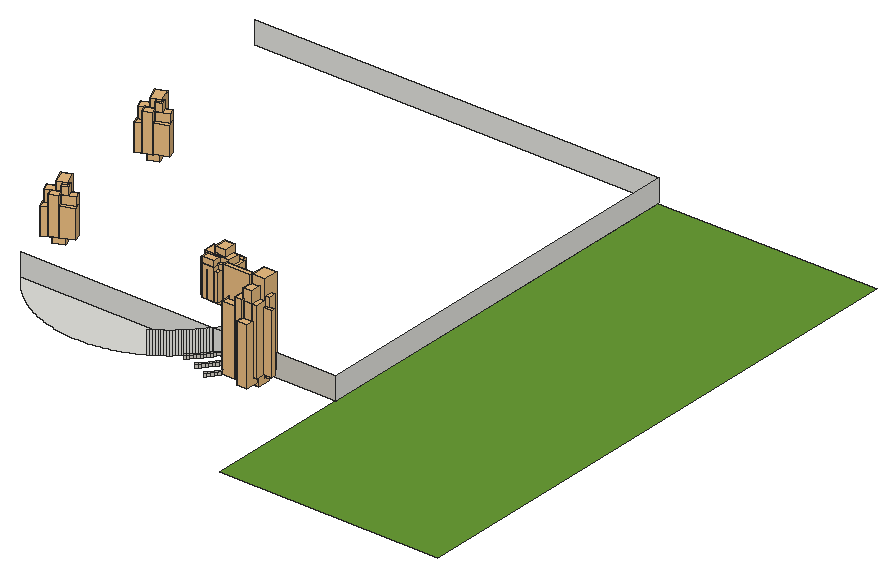
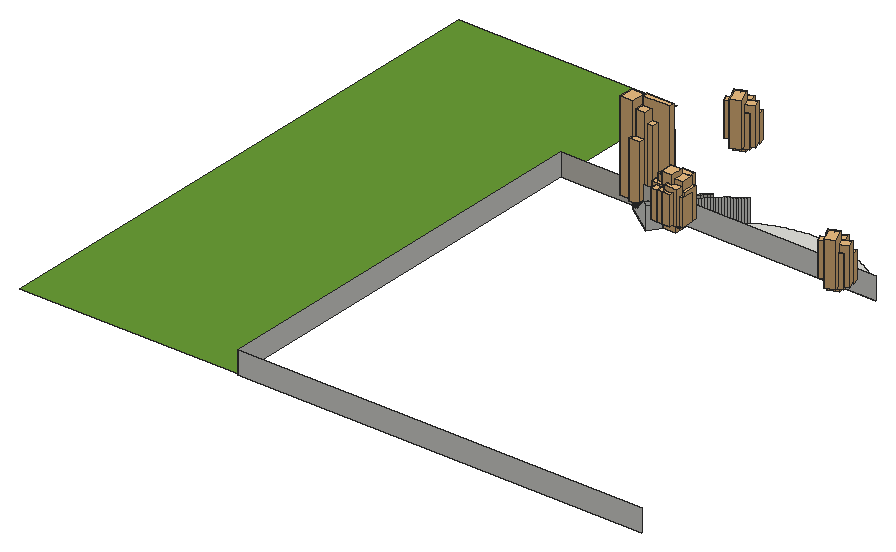
# SketchUp Ruby script. Lengths in inches.
U = 1.inch
M = Sketchup.active_model
def pt(a) = Geom::Point3d.new(a.map { |v| v * U })
def face(e, loops, mat)
  f = e.add_face(loops[0].map { |a| pt(a) })
  loops[1..].each { |l| e.add_face(l.map { |a| pt(a) }).erase! }
  f.material = f.back_material = mat if mat
  f
end
# faces: each face lists its corners as indices into pts; further lists are holes
def faces(e, pts, list, mat = nil) = list.each { |f| face(e, (f[0].is_a?(Array) ? f : [f]).map { |l| l.map { |i| pts[i] } }, mat) }
# xy, xz, yz: faces in a plane at the given z, y or x. An outline is a flat list of corners, or four numbers for a rectangle; further outlines are holes
def ring(l) = l.size == 4 ? [[l[0], l[1]], [l[2], l[1]], [l[2], l[3]], [l[0], l[3]]] : l.each_slice(2).to_a
def flat(e, list, mat, &to3) = list.each { |f| face(e, (f[0].is_a?(Array) ? f : [f]).map { |l| ring(l).map { |u, v| to3.(u, v) } }, mat) }
def xy(e, z, list, mat = nil) = flat(e, list, mat) { |x, y| [x, y, z] }
def xz(e, y, list, mat = nil) = flat(e, list, mat) { |x, z| [x, y, z] }
def yz(e, x, list, mat = nil) = flat(e, list, mat) { |y, z| [x, y, z] }
def lines(e, pts, list) = list.each { |a, b| e.add_line(pt(pts[a]), pt(pts[b])) }
# prism: a flat outline (further loops are holes) pulled along v
def prism(e, loops, v, mat = nil)
  f = face(e, loops, mat); d = Geom::Vector3d.new(v.map { |x| x * U })
  f.pushpull(f.normal.samedirection?(d) ? d.length : -d.length)
end
def box(e, o, s, mat = nil) = prism(e, [[o, [o[0] + s[0], o[1], o[2]], [o[0] + s[0], o[1] + s[1], o[2]], [o[0], o[1] + s[1], o[2]]]], [0, 0, s[2]], mat)
def at(x, y, z, deg = 0) = Geom::Transformation.translation(pt([x, y, z])) * Geom::Transformation.rotation(ORIGIN, Z_AXIS, deg.degrees)
def axes(o, x, y, z) = Geom::Transformation.new([*x, 0, *y, 0, *z, 0, *pt(o).to_a, 1])
def part(name) = M.definitions.add(name)
# library, detail: a bought-in or finely detailed component or shape, given as its bounding box
def library(name, o, s) = part(name).tap { |d| box(d.entities, o, s) }
def detail(e, o, s) = box(e.add_group.entities, o, s)
def put(e, d, t, mat = nil) = e.add_instance(d, t).tap { |i| i.material = mat if mat }
def group(e, t, mat = nil) = e.add_group.tap { |g| g.transformation = t; g.material = mat if mat }.entities
root = M.entities
M.materials.add("Arta-Ceramic-Moonstone-White-24x24-4K").color = [209, 205, 196]
M.materials.add("POT_TEXTURE_1").color = [172, 172, 172]
M.materials.add("[Grass Dark Green]").color = [106, 157, 55]
M.materials.add("soil1").color = [68, 55, 47]
M.materials.add("white_concrete_pot1").color = [212, 211, 204]
c1 = library("Group\#13",[-312.76,2118.02,370.79],[80.37,61.43,57.53])
c2 = library("Group\#34",[-146.29,2044.53,349.125],[81,53.32,37.9])
c3 = library("Group\#80",[-236.03,2064.57,238.29],[378.97,266.89,1422.96])
c4 = library("Group\#22",[-392.38,2142.99,345.23],[79.77,60.6,39.05])
c5 = library("Group\#49",[-390.04,2074.71,363.78],[77.3,84.83,61.55])
c6 = library("Group\#26",[-389.63,2051.04,359.41],[56.81,81.38,37.86])
c7 = library("Group\#30",[-362.86,1963.26,351.01],[55.56,80.44,37.9])
c8 = library("Group\#33",[-200.52,1998.86,370.22],[77.15,68.38,35.39])
c9 = library("Group\#45",[-480.58,1843.32,11.96],[467.85,466.24,378.92])
c10 = library("Group\#23",[-433.57,2042.61,369.7],[71.79,72.8,37.85])
c11 = library("Group\#20",[-148.5,2084.1,354.63],[73.89,71.73,39.48])
c12 = library("Group\#62",[-372.4375,2154.5,374],[76.125,67.08,39.0625])
c13 = library("Group\#63",[-275.5,2156.34,352.11],[71.39,73.27,44.69])
c14 = library("Group\#39",[-143.56,2061.14,371.42],[79.79,63.19,51.3])
c15 = library("Group\#48",[-363.89,1895.22,354.63],[76.92,66.54,39.48])
c16 = library("Group\#41",[-145.08,2015.32,369.99],[82.29,54.05,37.9])
c17 = library("Group\#59",[-315.77,2202.04,371],[80.74,54.44,37.85])
c18 = library("Group\#50",[-419.21,1941.11,355.02],[73.1,71.21,39.06])
c19 = library("Group\#53",[-229.79,1894.04,351.01],[79.82,63.55,37.9])
c20 = library("Group\#67",[-234.26,2180.97,367.05],[50.63,74.65,43.95])
c21 = library("Group\#69",[-904.81,1865.01,156.3],[624.43,217.34,1227.7])
c22 = library("Group\#70",[-312.51,1611.52,263.78],[120.52,408.52,1275.1])
c23 = library("Group\#71",[-571.16,1736.08,232.33],[294.08,306.57,1438.75])
c24 = library("Group\#73",[-273.21,1593.22,47.51],[374.54,419.07,1416.6])
c25 = library("Group\#17",[-202.35,1900.5,372.29],[58.53,80.11,50.06])
c26 = library("Group\#25",[-432.01,1984.38,372.6875],[64.1,75.95,39.0625])
c27 = library("Group\#38",[-310.7,1952.62,354.63],[79.53,58.52,39.48])
c28 = library("Group\#24",[-374.28,1979.7,369.99],[51.81,82.66,37.9])
c29 = library("Group\#56",[-397.18,1916.74,372.44],[70.02,74.57,49.25])
c30 = library("Group\#65",[-236.3,2186.8,344.47],[79.26,62.91,39.06])
c31 = library("Group\#16",[-161.07,2117.49,373.61],[81.25,53.73,39.48])
c32 = library("Group\#68",[-431.9,1883.46,368.72],[373.65,376.39,18.61])
c33 = library("Group\#37",[-340.96,1970.4,361.28],[81.22,51.59,61.62])
c34 = library("Group\#43",[-272.7,1884.51,369.99],[80.39,55.87,37.9])
c35 = library("Group\#32",[-330.83,2117.69,370.2],[61.83,80.2,35.55])
c36 = library("Group\#66",[-366.3125,2177.8,359.41],[79.9,61.23,37.86])
c37 = library("Group\#29",[-435.875,2067.96,347.82],[58.32,80.53,38.29])
c38 = library("Group\#64",[-183.79,2161.45,371.25],[72.43,70.21,54.35])
c39 = library("Group\#72",[-208.23,2037.18,75.37],[621.09,225.61,1251.82])
c40 = library("Group\#75",[-675.58,1862.05,152.55],[378.81,196.01,1743.84])
c41 = library("Group\#76",[-257.06,2048.08,160.05],[394.6,177.93,1743.83])
c42 = library("Group\#77",[-344.84,1500.61,160.55],[176.35,551.19,1921.45])
c43 = library("Group\#78",[-231.77,1913.24,119.96],[448.93,143.84,1582.05])
c44 = library("Group\#79",[-616.67,2098.6,178.29],[331.19,111.16,1177.92])
c45 = library("Group\#74",[-527.15,2088.47,150.96],[267.01,328.12,1599.25])
c46 = library("Group\#81",[-792.12,2067.32,152.13],[549.56,259.52,1931.8])
c47 = library("Group\#82",[-281.17,2118.67,243.77],[133.23,408.71,1313.3])
c48 = part("Tall potted plant")
g1 = group(c48.entities,at(904.81,-1500.61,-11.96),"white_concrete_pot1")
detail(g1,[-222.14,2117.95,372.07],[61.87,75.41,50.35])
put(c48.entities,c1,at(904.81,-1500.61,-11.96),"white_concrete_pot1")
g2 = group(c48.entities,at(904.81,-1500.61,-11.96),"white_concrete_pot1")
detail(g2,[-313.93,1881.02,351.21],[70.15,73.18,37.2])
g3 = group(c48.entities,at(904.81,-1500.61,-11.96),"white_concrete_pot1")
detail(g3,[-209.1,1970.26,378.89],[50.57,81.04,37.2])
put(c48.entities,c2,at(904.81,-1500.61,-11.96),"white_concrete_pot1")
put(c48.entities,c3,axes([904.81,-1500.61,-66.4],[1,0,0],[0,1,0],[0,0,2.14595]))
put(c48.entities,c4,at(904.81,-1500.61,-11.96),"white_concrete_pot1")
put(c48.entities,c5,at(904.81,-1500.61,-11.96),"white_concrete_pot1")
put(c48.entities,c6,at(904.81,-1500.61,-11.96),"white_concrete_pot1")
put(c48.entities,c7,at(904.81,-1500.61,-11.96),"white_concrete_pot1")
g4 = group(c48.entities,at(904.81,-1500.61,-11.96),"white_concrete_pot1")
detail(g4,[-129.49,1972.75,359.91],[55.59,80.76,37.2])
put(c48.entities,c8,at(904.81,-1500.61,-11.96),"white_concrete_pot1")
g5 = group(c48.entities,at(904.81,-1500.61,-11.96),"white_concrete_pot1")
detail(g5,[-333.13,1892.25,370.19],[61.39,79.4,37.2])
put(c48.entities,c9,at(904.81,-1500.61,-11.96),"POT_TEXTURE_1")
put(c48.entities,c10,at(904.81,-1500.61,-11.96),"white_concrete_pot1")
put(c48.entities,c11,at(904.81,-1500.61,-11.96),"white_concrete_pot1")
g6 = group(c48.entities,at(904.81,-1500.61,-11.96),"white_concrete_pot1")
detail(g6,[-270.91,2176.57,345.18],[52.11,82.01,38.29])
g7 = group(c48.entities,at(904.81,-1500.61,-11.96),"white_concrete_pot1")
detail(g7,[-195.71,2019.1875,371.11],[58.98,81.18,37.2])
g8 = group(c48.entities,at(904.81,-1500.61,-11.96),"white_concrete_pot1")
detail(g8,[-319.36,2078.81,339.18],[76.07,69.08,39.48])
put(c48.entities,c12,at(904.81,-1500.61,-11.96),"white_concrete_pot1")
put(c48.entities,c13,at(904.81,-1500.61,-11.96),"white_concrete_pot1")
g9 = group(c48.entities,at(904.81,-1500.61,-11.96),"white_concrete_pot1")
detail(g9,[-417.64,2112.53,369.82],[65.44,79.59,38.29])
put(c48.entities,c14,at(904.81,-1500.61,-11.96),"white_concrete_pot1")
put(c48.entities,c15,at(904.81,-1500.61,-11.96),"white_concrete_pot1")
put(c48.entities,c16,at(904.81,-1500.61,-11.96),"white_concrete_pot1")
g10 = group(c48.entities,at(904.81,-1500.61,-11.96),"white_concrete_pot1")
detail(g10,[-240.6,2054.85,378.89],[71.5,72.03,37.2])
put(c48.entities,c17,at(904.81,-1500.61,-11.96),"white_concrete_pot1")
put(c48.entities,c18,at(904.81,-1500.61,-11.96),"white_concrete_pot1")
put(c48.entities,c19,at(904.81,-1500.61,-11.96),"white_concrete_pot1")
g11 = group(c48.entities,at(904.81,-1500.61,-11.96),"white_concrete_pot1")
detail(g11,[-249.82,2117.53,359.91],[58.07,81.25,37.2])
put(c48.entities,c20,at(904.81,-1500.61,-11.96),"white_concrete_pot1")
put(c48.entities,c21,axes([904.81,-1500.61,-66.4],[1,0,0],[0,1,0],[0,0,2.14595]))
put(c48.entities,c22,axes([904.81,-1500.61,-66.4],[1,0,0],[0,1,0],[0,0,2.14595]))
put(c48.entities,c23,axes([904.81,-1500.61,-66.4],[1,0,0],[0,1,0],[0,0,2.14595]))
put(c48.entities,c24,axes([904.81,-1500.61,-66.4],[1,0,0],[0,1,0],[0,0,2.14595]))
g12 = group(c48.entities,at(904.81,-1500.61,-11.96),"white_concrete_pot1")
detail(g12,[-435.4375,2027.54,350.71],[78.74,62.6,37.86])
put(c48.entities,c25,at(904.81,-1500.61,-11.96),"white_concrete_pot1")
g13 = group(c48.entities,at(904.81,-1500.61,-11.96),"white_concrete_pot1")
detail(g13,[-173.8,2126.25,354.63],[80.17,60.53,39.48])
g14 = group(c48.entities,at(904.81,-1500.61,-11.96),"white_concrete_pot1")
detail(g14,[-222.96,2066.75,359.91],[63.77,78.21,37.2])
put(c48.entities,c26,at(904.81,-1500.61,-11.96),"white_concrete_pot1")
g15 = group(c48.entities,at(904.81,-1500.61,-11.96),"white_concrete_pot1")
detail(g15,[-183.125,1913.38,330.04],[66.78,77.69,39.48])
put(c48.entities,c27,at(904.81,-1500.61,-11.96),"white_concrete_pot1")
g16 = group(c48.entities,at(904.81,-1500.61,-11.96),"white_concrete_pot1")
detail(g16,[-152,1936.85,378.89],[64.46,79.76,37.2])
g17 = group(c48.entities,at(904.81,-1500.61,-11.96),"white_concrete_pot1")
detail(g17,[-284.65,1933.22,373.64],[80.83,55.23,37.2])
put(c48.entities,c28,at(904.81,-1500.61,-11.96),"white_concrete_pot1")
g18 = group(c48.entities,at(904.81,-1500.61,-11.96),"white_concrete_pot1")
detail(g18,[-263.49,1923.54,359.91],[75.98,66.75,37.2])
put(c48.entities,c29,at(904.81,-1500.61,-11.96),"white_concrete_pot1")
g19 = group(c48.entities,at(904.81,-1500.61,-11.96),"white_concrete_pot1")
detail(g19,[-167.97,1940.97,354.63],[66.78,77.7,39.48])
put(c48.entities,c30,at(904.81,-1500.61,-11.96),"white_concrete_pot1")
g20 = group(c48.entities,at(904.81,-1500.61,-11.96),"white_concrete_pot1")
detail(g20,[-214.75,1956.59,330.04],[66.78,77.69,39.48])
put(c48.entities,c31,at(904.81,-1500.61,-11.96),"white_concrete_pot1")
put(c48.entities,c32,at(904.81,-1500.61,-11.96),"white_concrete_pot1")
put(c48.entities,c33,at(904.81,-1500.61,-11.96),"white_concrete_pot1")
g21 = group(c48.entities,at(904.81,-1500.61,-11.96),"white_concrete_pot1")
detail(g21,[-282.5625,1934.21,389.56],[81.1,59.19,35.03])
put(c48.entities,c34,at(904.81,-1500.61,-11.96),"white_concrete_pot1")
g22 = group(c48.entities,at(904.81,-1500.61,-11.96),"white_concrete_pot1")
detail(g22,[-394.5,2036.48,359.91],[79.58,64.84,37.2])
put(c48.entities,c35,at(904.81,-1500.61,-11.96),"white_concrete_pot1")
put(c48.entities,c36,at(904.81,-1500.61,-11.96),"white_concrete_pot1")
put(c48.entities,c37,at(904.81,-1500.61,-11.96),"white_concrete_pot1")
put(c48.entities,c38,at(904.81,-1500.61,-11.96),"white_concrete_pot1")
put(c48.entities,c39,axes([904.81,-1500.61,-66.4],[1,0,0],[0,1,0],[0,0,2.14595]))
put(c48.entities,c40,axes([904.81,-1500.61,-66.4],[1,0,0],[0,1,0],[0,0,2.14595]))
put(c48.entities,c41,axes([904.81,-1500.61,-66.4],[1,0,0],[0,1,0],[0,0,2.14595]))
put(c48.entities,c42,axes([904.81,-1500.61,-66.4],[1,0,0],[0,1,0],[0,0,2.14595]))
put(c48.entities,c43,axes([904.81,-1500.61,-66.4],[1,0,0],[0,1,0],[0,0,2.14595]))
put(c48.entities,c44,axes([904.81,-1500.61,-66.4],[1,0,0],[0,1,0],[0,0,2.14595]))
put(c48.entities,c45,axes([904.81,-1500.61,-66.4],[1,0,0],[0,1,0],[0,0,2.14595]))
put(c48.entities,c46,axes([904.81,-1500.61,-66.4],[1,0,0],[0,1,0],[0,0,2.14595]))
put(c48.entities,c47,axes([904.81,-1500.61,-66.4],[1,0,0],[0,1,0],[0,0,2.14595]))
c49 = library("Group\#90",[-662.41,217.3,320.04],[397.32,658.3,1732.06])
c50 = library("Group\#92",[-299.2,181.55,262.58],[360.65,735.71,1258.34])
c51 = library("Group\#87",[-1038.76,656.55,345.34],[733.18,460.51,2065.7])
c52 = library("Group\#85",[-445.29,890.31,329.28],[284.3,304.08,2023.29])
c53 = library("Group\#88",[-733.48,439.625,202.64],[456.28,533.12,1536.78])
c54 = library("Group\#91",[-455.56,899.32,410.78],[341.21,610.33,1581.5])
c55 = library("Group\#84",[-516.34,626.77,-4.5625],[517.73,515.95,418.98])
c56 = library("Group\#89",[-249.24,914.85,310.18],[345.55,647.95,1307.93])
c57 = library("Group\#86",[-277.97,488.68,287.26],[362.84,405.94,1768.54])
c58 = library("Group\#83",[-468.76,669.89,380.1875],[424.36,427.47,41.99])
c59 = part("Potted broadleaf plant")
put(c59.entities,c49,at(1038.76,-181.55,4.5625))
put(c59.entities,c50,at(1038.76,-181.55,4.5625))
put(c59.entities,c51,at(1038.76,-181.55,4.5625))
put(c59.entities,c52,at(1038.76,-181.55,4.5625))
put(c59.entities,c53,at(1038.76,-181.55,4.5625))
put(c59.entities,c54,at(1038.76,-181.55,4.5625))
put(c59.entities,c55,at(1038.76,-181.55,4.5625),"POT_TEXTURE_1")
put(c59.entities,c56,at(1038.76,-181.55,4.5625))
put(c59.entities,c57,at(1038.76,-181.55,4.5625))
put(c59.entities,c58,at(1038.76,-181.55,4.5625),"soil1")
c60 = library("Group\#131",[-640.625,-1318.37,287.11],[396.64,314.81,689.96])
c61 = library("Group\#123",[-513.94,-1201.2,195.17],[480.66,557.42,1160.08])
c62 = library("Group\#128",[-208.03,-1336.63,286.21],[381.72,484.79,1145.39])
c63 = library("Group\#134",[-619.83,-1636.3,288.9],[316.15,456.61,1171.28])
c64 = library("Group\#135",[-738.91,-1210.08,301],[426.4,388.88,1000.79])
c65 = library("Group\#137",[-208.33,-1511.76,297.04],[508.2,421.96,1258.76])
c66 = library("Group\#127",[-545.36,-1775.03,287.125],[412.21,432,920.68])
c67 = library("Group\#132",[-750.24,-1478.51,301.56],[423.84,451.05,998.69])
c68 = library("Group\#130",[-245.33,-1174.2,301.22],[356.02,306.31,608.34])
c69 = library("Group\#122",[-487.23,-1483.58,-4.71],[450.86,446.99,418.38])
c70 = library("Group\#139",[-445.7,-1606.55,154.18],[255.44,283.57,849.28])
c71 = library("Group\#140",[-390.1,-1177.12,195.59],[220.93,265.44,790.12])
c72 = library("Group\#142",[-480.32,-1333.42,295.8],[424.49,356.06,1482.77])
c73 = library("Group\#143",[-378.01,-1245.98,305.66],[422.15,474.55,1267.42])
c74 = library("Group\#129",[-163.65,-1622.09,292.29],[406.18,374.8,780.12])
c75 = library("Group\#138",[-384.8,-1640.99,300.61],[422.68,348.03,1297.96])
c76 = library("Group\#121",[-429.18,-1441.17,362.05],[345.84,348.28,45.35])
c77 = library("Group\#141",[-208.0625,-1498.77,286.27],[547.26,435.76,1075.6])
c78 = library("Group\#136",[-172.82,-1329.68,294.68],[502.85,397.72,955.79])
c79 = library("Group\#133",[-426.76,-1753.59,287.48],[479.67,412.35,1049.19])
c80 = part("Potted palm")
put(c80.entities,c60,at(750.24,1775.03,4.71))
put(c80.entities,c61,at(750.24,1775.03,4.71))
put(c80.entities,c62,at(750.24,1775.03,4.71))
put(c80.entities,c63,at(750.24,1775.03,4.71))
put(c80.entities,c64,at(750.24,1775.03,4.71))
put(c80.entities,c65,at(750.24,1775.03,4.71))
put(c80.entities,c66,at(750.24,1775.03,4.71))
put(c80.entities,c67,at(750.24,1775.03,4.71))
put(c80.entities,c68,at(750.24,1775.03,4.71))
put(c80.entities,c69,at(750.24,1775.03,4.71),"POT_TEXTURE_1")
put(c80.entities,c70,at(750.24,1775.03,4.71))
put(c80.entities,c71,at(750.24,1775.03,4.71))
put(c80.entities,c72,at(750.24,1775.03,4.71))
put(c80.entities,c73,at(750.24,1775.03,4.71))
put(c80.entities,c74,at(750.24,1775.03,4.71))
put(c80.entities,c75,at(750.24,1775.03,4.71))
put(c80.entities,c76,at(750.24,1775.03,4.71),"soil1")
put(c80.entities,c77,at(750.24,1775.03,4.71))
put(c80.entities,c78,at(750.24,1775.03,4.71))
put(c80.entities,c79,at(750.24,1775.03,4.71))
c81 = part("plants(3)")
put(c81.entities,c48,axes([-11089.18,3571.64,160.04],[1.28,0,0],[0,2.25883,0],[0,0,1]))
put(c81.entities,c59,at(-12958.47,-6842.38,1209,22))
put(c81.entities,c80,axes([-13314.6875,820.47,1209],[1.33,0,0],[0,1.33,0],[0,0,1.33]))
put(c81.entities,c59,at(-13453.34,-2834.26,5889.94,22))
xy(root,0,[[1024.28,128.0625,1021.27,128.09,1018.26,128.18,1015.26,128.32,1012.25,128.52,1009.26,128.78,1006.26,129.1,1003.28,129.48,1000.3,129.91,997.33,130.4,994.37,130.94,991.42,131.54,988.48,132.2,985.56,132.92,982.65,133.6875,979.76,134.51,976.88,135.4,974.02,136.33,971.18,137.32,968.36,138.37,965.56,139.47,962.78,140.625,960.02,141.83,957.28,143.09,954.58,144.4,951.89,145.76,949.24,147.18,946.61,148.64,944.01,150.16,941.4375,151.72,938.9,153.34,936.39,155,933.91,156.71,931.47,158.47,929.06,160.27,926.69,162.12,924.35,164.02,922.05,165.96,919.78,167.94,917.56,169.97,915.37,172.04,913.23,174.15,911.12,176.3,909.06,178.49,907.04,180.72,905.06,182.99,903.125,185.29,901.24,187.64,899.39,190.01,897.59,192.43,895.84,194.875,1152.72,194.875,1150.97,192.43,1149.17,190.01,1147.33,187.64,1145.4375,185.29,1143.5,182.99,1141.52,180.72,1139.5,178.49,1137.44,176.3,1135.34,174.15,1133.19,172.04,1131,169.97,1128.78,167.94,1126.52,165.96,1124.21,164.02,1121.875,162.12,1119.5,160.27,1117.09,158.47,1114.65,156.71,1112.17,155,1109.67,153.34,1107.125,151.72,1104.55,150.16,1101.95,148.64,1099.33,147.18,1096.67,145.76,1093.99,144.4,1091.28,143.09,1088.54,141.83,1085.79,140.625,1083.01,139.47,1080.21,138.37,1077.38,137.32,1074.54,136.33,1071.68,135.4,1068.8,134.51,1065.91,133.6875,1063,132.92,1060.08,132.2,1057.14,131.54,1054.19,130.94,1051.23,130.4,1048.26,129.91,1045.28,129.48,1042.3,129.1,1039.31,128.78,1036.31,128.52,1033.3,128.32,1030.3,128.18,1027.29,128.09],[1152.72,194.875,1177.16,229.03,1216.84,200.64,1212.72,194.875],[1318.125,194.875,1318.21,733.875]])
xy(root,0,[[1318.125,0,1318.125,194.875,1318.21,194.875,1318.21,733.875,1610.5625,733.875,1610.5625,0]],"[Grass Dark Green]")
xy(root,6,[[1200.72,194.875,1212.72,194.875,1216.84,200.64,1208.91,206.32]])
xy(root,12,[[1188.72,194.875,1200.72,194.875,1201.05,195.33,1208.91,206.32,1200.97,212]])
xz(root,194.875,[[895.84,0,1152.72,30],[1152.72,0,1212.72,0,1212.72,6,1200.72,6,1200.72,12,1188.72,12,1188.72,18,1176.72,18,1176.72,24,1164.72,24,1164.72,30,1152.72,30]])
xz(root,194.875,[[1212.72,0,1318.21,0,1318.21,30,1164.72,30,1164.72,24,1176.72,24,1176.72,18,1188.72,18,1188.72,12,1200.72,12,1200.72,6,1212.72,6]],"Arta-Ceramic-Moonstone-White-24x24-4K")
xz(root,734.875,[[777.4375,0,1318.21,30]])
yz(root,1318.21,[[194.875,0,734.875,30]])
p = [[1178,148.3,5],[1178,148.3,0],[1180.59,151.27,0],[1180.59,151.27,5],[1101.95,148.64,0],[1101.95,148.64,30],
  [1104.55,150.16,30],[1104.55,150.16,0],[1107.125,151.72,30],[1107.125,151.72,0],[1183.13,154.3,0],[1183.13,154.3,5],
  [1109.67,153.34,30],[1109.67,153.34,0],[1112.17,155,30],[1112.17,155,0],[1185.6,157.37,0],[1185.6,157.37,5],
  [1114.65,156.71,30],[1114.65,156.71,0],[1117.09,158.47,30],[1117.09,158.47,0],[1188.02,160.49,0],[1188.02,160.49,5],
  [1119.5,160.27,30],[1119.5,160.27,0],[1121.875,162.12,30],[1121.875,162.12,0],[1190.38,163.65,0],[1190.38,163.65,5],
  [1124.21,164.02,30],[1124.21,164.02,0],[1212.72,194.875,0],[1212.72,194.875,5],[1126.52,165.96,30],[1126.52,165.96,0],
  [1128.78,167.94,30],[1128.78,167.94,0],[1131,169.97,30],[1131,169.97,0],[1133.19,172.04,30],[1133.19,172.04,0],
  [1135.34,174.15,30],[1135.34,174.15,0],[1137.44,176.3,30],[1137.44,176.3,0],[1139.5,178.49,30],[1139.5,178.49,0],
  [1141.52,180.72,30],[1141.52,180.72,0],[1143.5,182.99,30],[1143.5,182.99,0],[1145.4375,185.29,30],[1145.4375,185.29,0],
  [1147.33,187.64,30],[1147.33,187.64,0],[1149.17,190.01,30],[1149.17,190.01,0],[1150.97,192.43,30],[1150.97,192.43,0],
  [1152.72,194.875,0],[1152.72,194.875,30],[1177.16,229.03,0],[1177.16,229.03,30],[1216.84,200.64,6],[1212.72,194.875,6],
  [1216.84,200.64,0],[1208.91,206.32,6],[1185.09,223.35,30],[1185.09,223.35,24],[1193.03,217.67,24],[1193.03,217.67,18],
  [1200.97,212,18],[1200.97,212,12],[1208.91,206.32,12],[1178.61,147.76,6],[1178.61,147.76,5],[1181.21,150.75,5],
  [1181.21,150.75,6],[1183.76,153.78,5],[1183.76,153.78,6],[1186.24,156.87,5],[1186.24,156.87,6],[1188.67,160,5],
  [1188.67,160,6],[1191.04,163.17,5],[1191.04,163.17,6],[1213.38,194.4,5],[1213.38,194.4,6],[1165.6,149.26,11],
  [1165.6,149.26,6],[1168.18,152,6],[1168.18,152,11],[1170.7,154.78,6],[1170.7,154.78,11],[1173.17,157.62,6],
  [1173.17,157.62,11],[1175.59,160.5,6],[1175.59,160.5,11],[1177.95,163.42,6],[1177.95,163.42,11],[1180.25,166.39,6],
  [1180.25,166.39,11],[1182.5,169.41,6],[1182.5,169.41,11],[1200.72,194.875,6],[1200.72,194.875,11],[1201.05,195.33,12],
  [1201.05,195.33,11],[1166.19,148.7,12],[1166.19,148.7,11],[1168.78,151.45,11],[1168.78,151.45,12],[1171.3125,154.24,11],
  [1171.3125,154.24,12],[1173.79,157.09,11],[1173.79,157.09,12],[1176.22,159.98,11],[1176.22,159.98,12],[1178.59,162.92,11],
  [1178.59,162.92,12],[1180.9,165.9,11],[1180.9,165.9,12],[1183.15,168.93,11],[1183.15,168.93,12],[1201.71,194.86,11],
  [1201.71,194.86,12],[1200.72,194.875,12],[1150.93,148.51,17],[1150.93,148.51,12],[1153.52,150.96,12],[1153.52,150.96,17],
  [1156.07,153.47,12],[1156.07,153.47,17],[1158.5625,156.02,12],[1158.5625,156.02,17],[1161.01,158.62,12],[1161.01,158.62,17],
  [1163.41,161.27,12],[1163.41,161.27,17],[1165.76,163.96,12],[1165.76,163.96,17],[1168.05,166.7,12],[1168.05,166.7,17],
  [1170.29,169.48,12],[1170.29,169.48,17],[1172.48,172.3,12],[1172.48,172.3,17],[1174.61,175.16,12],[1174.61,175.16,17],
  [1188.72,194.875,12],[1188.72,194.875,17],[1189.08,195.38,18],[1189.08,195.38,17],[1151.48,147.91,18],[1151.48,147.91,17],
  [1154.08,150.38,17],[1154.08,150.38,18],[1156.64,152.89,17],[1156.64,152.89,18],[1159.15,155.46,17],[1159.15,155.46,18],
  [1161.61,158.07,17],[1161.61,158.07,18],[1164.02,160.73,17],[1164.02,160.73,18],[1166.375,163.43,17],[1166.375,163.43,18],
  [1168.68,166.18,17],[1168.68,166.18,18],[1170.93,168.97,17],[1170.93,168.97,18],[1173.13,171.81,17],[1173.13,171.81,18],
  [1175.27,174.68,17],[1175.27,174.68,18],[1189.74,194.91,17],[1189.74,194.91,18],[1188.72,194.875,18]]
faces(root,p,[[0,1,2,3],[3,2,10,11],[11,10,16,17],[17,16,22,23],[23,22,28,29],[28,32,33,29],[75,76,77,78],[78,77,79,80],
  [80,79,81,82],[82,81,83,84],[84,83,85,86],[86,85,87,88],[87,33,65,88],[89,90,91,92],[92,91,93,94],[94,93,95,96],
  [96,95,97,98],[98,97,99,100],[100,99,101,102],[102,101,103,104],[103,105,106,104],[109,110,111,112],[112,111,113,114],[114,113,115,116],
  [116,115,117,118],[118,117,119,120],[120,119,121,122],[122,121,123,124],[124,123,125,126],[127,106,108,107],[125,108,107,126],[128,129,130,131],
  [131,130,132,133],[133,132,134,135],[135,134,136,137],[137,136,138,139],[139,138,140,141],[141,140,142,143],[143,142,144,145],[145,144,146,147],
  [147,146,148,149],[148,150,151,149],[154,155,156,157],[157,156,158,159],[159,158,160,161],[161,160,162,163],[163,162,164,165],[165,164,166,167],
  [167,166,168,169],[169,168,170,171],[171,170,172,173],[173,172,174,175],[175,174,176,177],[178,151,153,152],[176,153,152,177]],"Arta-Ceramic-Moonstone-White-24x24-4K")
faces(root,p,[[4,5,6,7],[7,6,8,9],[9,8,12,13],[13,12,14,15],[15,14,18,19],[19,18,20,21],[21,20,24,25],[25,24,26,27],
  [27,26,30,31],[31,30,34,35],[35,34,36,37],[37,36,38,39],[39,38,40,41],[41,40,42,43],[43,42,44,45],[45,44,46,47],
  [47,46,48,49],[49,48,50,51],[51,50,52,53],[53,52,54,55],[55,54,56,57],[57,56,58,59],[60,59,58,61],[62,60,61,63],
  [64,65,33,32,66],[67,64,66,62,63,68,69,70,71,72,73,74],[74,107,108,106,105,67],[72,152,153,151,150,73]])
put(root,c81,axes([1081.79,-116.37,-4.58],[0,-0.0286,0],[0.0286,0,0],[0,0,0.0286]))
